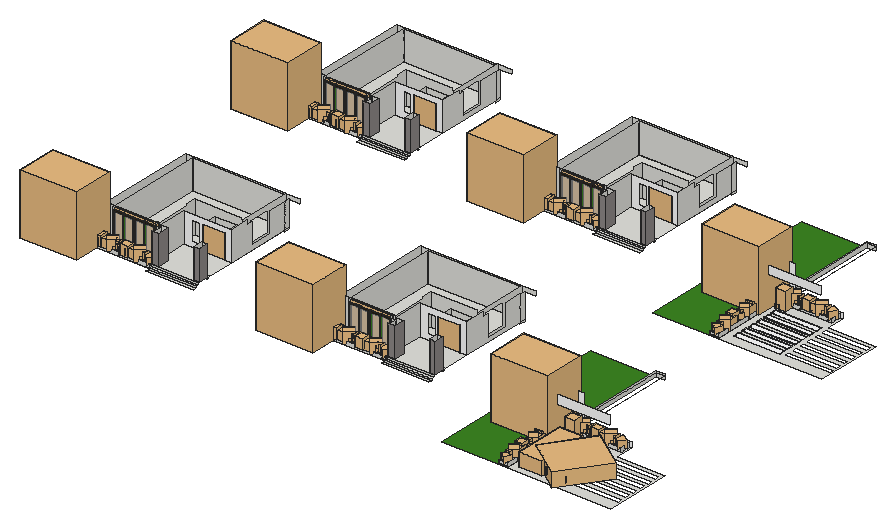
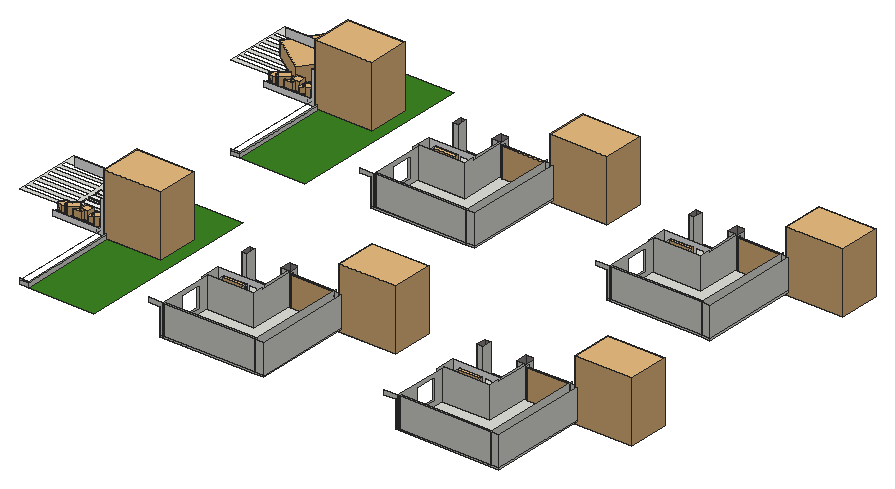
# SketchUp Ruby script. Lengths in inches.
U = 1.inch
M = Sketchup.active_model
def pt(a) = Geom::Point3d.new(a.map { |v| v * U })
def face(e, loops, mat)
  f = e.add_face(loops[0].map { |a| pt(a) })
  loops[1..].each { |l| e.add_face(l.map { |a| pt(a) }).erase! }
  f.material = f.back_material = mat if mat
  f
end
# faces: each face lists its corners as indices into pts; further lists are holes
def faces(e, pts, list, mat = nil) = list.each { |f| face(e, (f[0].is_a?(Array) ? f : [f]).map { |l| l.map { |i| pts[i] } }, mat) }
# xy, xz, yz: faces in a plane at the given z, y or x. An outline is a flat list of corners, or four numbers for a rectangle; further outlines are holes
def ring(l) = l.size == 4 ? [[l[0], l[1]], [l[2], l[1]], [l[2], l[3]], [l[0], l[3]]] : l.each_slice(2).to_a
def flat(e, list, mat, &to3) = list.each { |f| face(e, (f[0].is_a?(Array) ? f : [f]).map { |l| ring(l).map { |u, v| to3.(u, v) } }, mat) }
def xy(e, z, list, mat = nil) = flat(e, list, mat) { |x, y| [x, y, z] }
def xz(e, y, list, mat = nil) = flat(e, list, mat) { |x, z| [x, y, z] }
def yz(e, x, list, mat = nil) = flat(e, list, mat) { |y, z| [x, y, z] }
def lines(e, pts, list) = list.each { |a, b| e.add_line(pt(pts[a]), pt(pts[b])) }
# prism: a flat outline (further loops are holes) pulled along v
def prism(e, loops, v, mat = nil)
  f = face(e, loops, mat); d = Geom::Vector3d.new(v.map { |x| x * U })
  f.pushpull(f.normal.samedirection?(d) ? d.length : -d.length)
end
def box(e, o, s, mat = nil) = prism(e, [[o, [o[0] + s[0], o[1], o[2]], [o[0] + s[0], o[1] + s[1], o[2]], [o[0], o[1] + s[1], o[2]]]], [0, 0, s[2]], mat)
def at(x, y, z, deg = 0) = Geom::Transformation.translation(pt([x, y, z])) * Geom::Transformation.rotation(ORIGIN, Z_AXIS, deg.degrees)
def axes(o, x, y, z) = Geom::Transformation.new([*x, 0, *y, 0, *z, 0, *pt(o).to_a, 1])
def part(name) = M.definitions.add(name)
# library, detail: a bought-in or finely detailed component or shape, given as its bounding box
def library(name, o, s) = part(name).tap { |d| box(d.entities, o, s) }
def detail(e, o, s) = box(e.add_group.entities, o, s)
def put(e, d, t, mat = nil) = e.add_instance(d, t).tap { |i| i.material = mat if mat }
def group(e, t, mat = nil) = e.add_group.tap { |g| g.transformation = t; g.material = mat if mat }.entities
root = M.entities
M.materials.add("Material__1").color = [95, 70, 46]
M.materials.add("[Carrera Marble]").color = [255, 255, 255]
M.materials.add("[Color M00]").color = [255, 255, 255]
M.materials.add("[Color M04]").color = [60, 133, 34]
M.materials.add("[Stone Marble]1").color = [143, 138, 136]
M.materials.add("[Translucent Glass Gray]2").color = [201, 201, 201]
M.materials["[Translucent Glass Gray]2"].alpha = 0.5
M.materials.add("[Wood Veneer 01]").color = [76, 44, 23]
M.materials.add("oak swatch").color = [40, 31, 19]
c1 = library("Group\#18",[0,0,0],[68.35,49.34,73.02])
c2 = library("Areca palm plant",[0,0,0],[49.1,36.6,54.46])
c3 = library("Group\#14",[-84.69,-90.07,-0.36],[176.51,175.13,171.4])
c4 = part("Group\#15")
xy(c4.entities,0,[[0,0,6,234.8],[30,0,36,234.8]])
xy(c4.entities,3,[[6,0,30,234.8]])
xy(c4.entities,7,[[6,5,30,229.8]],"Material__1")
xy(c4.entities,15,[[[0,0,36,234.8],[6,5,30,229.8]]])
xz(c4.entities,0,[[0,0,6,0,6,3,30,3,30,0,36,0,36,15,0,15]])
xz(c4.entities,5,[[6,7,30,15]])
xz(c4.entities,229.8,[[6,7,30,15]])
xz(c4.entities,234.8,[[0,0,0,15,36,15,36,0,30,0,30,3,6,3,6,0]])
yz(c4.entities,0,[[0,0,234.8,15]])
yz(c4.entities,6,[[0,0,234.8,3],[5,7,229.8,15]])
yz(c4.entities,30,[[0,0,234.8,3],[5,7,229.8,15]])
yz(c4.entities,36,[[0,0,234.8,15]])
c5 = library("Group20\#1",[-20.81,-17.08,3.79],[39.86,39.43,37.51])
c6 = library("Group38\#2",[14.01,28.44,-23.43],[18.58,18.32,38.89])
c7 = library("Group\#130",[-7.34,-1.2,0],[38.67,35.81,49.04])
c8 = part("Group\#16")
put(c8.entities,c2,axes([-6.2,158.41,6.08],[0.45017,-0.56191,0],[0.66137,0.52986,0],[0,0,0.72]))
put(c8.entities,c2,axes([-6.2,56.6,6.08],[0.45017,-0.56191,0],[0.66137,0.52986,0],[0,0,0.72]))
put(c8.entities,c3,axes([14.93,91.37,6.05],[-0.04961,-0.08593,0],[0.08593,-0.04961,0],[0,0,0.10522]))
put(c8.entities,c3,axes([14.93,145.87,6.05],[-0.04961,-0.08593,0],[0.08593,-0.04961,0],[0,0,0.10522]))
put(c8.entities,c3,axes([17.19,223.04,6.07],[-0.08133,-0.14087,0],[0.14087,-0.08133,0],[0,0,0.1725]))
put(c8.entities,c4,at(0,0,0))
put(c8.entities,c3,axes([14.93,193.18,6.05],[-0.04961,-0.08593,0],[0.08593,-0.04961,0],[0,0,0.10522]))
put(c8.entities,c3,axes([17.19,15.79,6.07],[-0.08133,-0.14087,0],[0.14087,-0.08133,0],[0,0,0.1725]))
put(c8.entities,c5,axes([18.97,181.79,4.77],[0,0.85,0],[-0.85,0,0],[0,0,0.85]))
put(c8.entities,c5,axes([18.97,79.98,4.77],[0,0.85,0],[-0.85,0,0],[0,0,0.85]))
put(c8.entities,c6,axes([-4.1,-1.15,28.17],[0.8848,0,0],[0,0.94674,0],[0,0,0.85826]))
put(c8.entities,c6,axes([-4.1,100.66,28.17],[0.8848,0,0],[0,0.94674,0],[0,0,0.85826]))
put(c8.entities,c7,axes([24.9375,89.91,8],[0,0.79,0],[-0.79,0,0],[0,0,0.79]))
put(c8.entities,c3,axes([14.93,173.12,6.05],[-0.04961,-0.08593,0],[0.08593,-0.04961,0],[0,0,0.10522]))
put(c8.entities,c3,axes([14.93,44.05,6.05],[-0.04961,-0.08593,0],[0.08593,-0.04961,0],[0,0,0.10522]))
put(c8.entities,c3,axes([14.93,71.3,6.05],[-0.04961,-0.08593,0],[0.08593,-0.04961,0],[0,0,0.10522]))
put(c8.entities,c7,axes([24.9375,191.72,8],[0,0.79,0],[-0.79,0,0],[0,0,0.79]))
put(c8.entities,c3,axes([17.19,121.23,6.07],[-0.08133,-0.14087,0],[0.14087,-0.08133,0],[0,0,0.1725]))
c9 = library("Curtains",[0,0,0],[121.73,8.19,117.22])
c10 = part("Group\#6")
box(c10.entities,[0,0,0],[1.77,4.72,80.31],"oak swatch")
c11 = part("Exterior Sliding Doors")
xy(c11.entities,0,[[1.77,33.07,3.54,70.87],[1.77,70.87,3.54,108.66]])
xy(c11.entities,0,[[0,0,1.77,33.07],[0,108.66,1.77,141.73]],"oak swatch")
xy(c11.entities,4.72,[[0,4.72,1.77,33.07],[1.77,37.8,3.54,66.14],[1.77,75.88,3.54,103.9375],[0,108.66,1.77,137.01]],"oak swatch")
xy(c11.entities,75.59,[[1.77,37.8,3.54,66.14],[1.77,75.88,3.54,103.9375]])
xy(c11.entities,75.59,[[0,4.72,1.77,33.07],[0,108.66,1.77,137.01]],"oak swatch")
xy(c11.entities,80.31,[[0,0,1.77,33.07],[1.77,33.07,3.54,70.87],[1.77,70.87,3.54,108.66],[0,108.66,1.77,141.73]],"oak swatch")
xz(c11.entities,0,[[0,0,1.77,80.31]],"oak swatch")
xz(c11.entities,4.72,[[0,4.72,1.77,75.59]],"oak swatch")
xz(c11.entities,33.07,[[0,0,1.77,4.72],[1.77,0,3.54,80.31],[0,75.59,1.77,80.31]],"oak swatch")
xz(c11.entities,37.8,[[1.77,4.72,3.54,75.59]])
xz(c11.entities,66.14,[[1.77,4.72,3.54,75.59]],"oak swatch")
xz(c11.entities,70.87,[[1.77,0,3.54,80.31]])
xz(c11.entities,75.88,[[1.77,4.72,3.54,75.59]])
xz(c11.entities,103.9375,[[1.77,4.72,3.54,75.59]],"oak swatch")
xz(c11.entities,108.66,[[1.77,4.72,3.54,75.59]])
xz(c11.entities,108.66,[[0,0,3.54,4.72],[0,75.59,3.54,80.31]],"oak swatch")
xz(c11.entities,137.01,[[0,4.72,1.77,75.59]],"oak swatch")
xz(c11.entities,141.73,[[0,0,1.77,80.31]],"oak swatch")
yz(c11.entities,0,[[0,0,33.07,0,33.07,4.72,4.72,4.72,4.72,75.59,33.07,75.59,33.07,80.31,0,80.31],[108.66,0,141.73,0,141.73,80.31,108.66,80.31,108.66,75.59,137.01,75.59,137.01,4.72,108.66,4.72]],"oak swatch")
yz(c11.entities,1.77,[[4.72,4.72,33.07,75.59],[37.8,4.72,66.14,75.59],[75.88,4.72,103.9375,75.59],[108.66,4.72,137.01,75.59]],"[Translucent Glass Gray]2")
yz(c11.entities,1.77,[[0,0,33.07,0,33.07,4.72,4.72,4.72,4.72,75.59,33.07,75.59,33.07,80.31,0,80.31],[[33.07,0,70.87,80.31],[37.8,4.72,66.14,75.59]],[[70.87,0,141.73,80.31],[108.66,4.72,137.01,75.59],[75.88,4.72,103.9375,75.59]]],"oak swatch")
yz(c11.entities,3.54,[[[33.07,0,70.87,80.31],[37.8,4.72,66.14,75.59]],[[70.87,0,108.66,80.31],[75.88,4.72,103.9375,75.59]]],"oak swatch")
put(c11.entities,c10,at(0,33.07,0))
put(c11.entities,c10,at(0,103.9375,0))
c12 = library("modern+door",[0,0,0],[59.06,11.8125,86.61])
c13 = part("Group\#17")
put(c13.entities,c2,axes([-6.2,56.6,6.08],[0.45017,-0.56191,0],[0.66137,0.52986,0],[0,0,0.72]))
put(c13.entities,c2,axes([-6.2,158.41,6.08],[0.45017,-0.56191,0],[0.66137,0.52986,0],[0,0,0.72]))
put(c13.entities,c3,axes([14.93,44.05,6.05],[-0.04961,-0.08593,0],[0.08593,-0.04961,0],[0,0,0.10522]))
put(c13.entities,c3,axes([14.93,71.3,6.05],[-0.04961,-0.08593,0],[0.08593,-0.04961,0],[0,0,0.10522]))
put(c13.entities,c5,axes([18.97,79.98,4.77],[0,0.85,0],[-0.85,0,0],[0,0,0.85]))
put(c13.entities,c3,axes([14.93,145.87,6.05],[-0.04961,-0.08593,0],[0.08593,-0.04961,0],[0,0,0.10522]))
put(c13.entities,c3,axes([17.19,15.79,6.07],[-0.08133,-0.14087,0],[0.14087,-0.08133,0],[0,0,0.1725]))
put(c13.entities,c3,axes([17.19,223.04,6.07],[-0.08133,-0.14087,0],[0.14087,-0.08133,0],[0,0,0.1725]))
put(c13.entities,c3,axes([17.19,121.23,6.07],[-0.08133,-0.14087,0],[0.14087,-0.08133,0],[0,0,0.1725]))
put(c13.entities,c7,axes([24.9375,191.72,8],[0,0.79,0],[-0.79,0,0],[0,0,0.79]))
put(c13.entities,c7,axes([24.9375,89.91,8],[0,0.79,0],[-0.79,0,0],[0,0,0.79]))
put(c13.entities,c3,axes([14.93,91.37,6.05],[-0.04961,-0.08593,0],[0.08593,-0.04961,0],[0,0,0.10522]))
put(c13.entities,c5,axes([18.97,181.79,4.77],[0,0.85,0],[-0.85,0,0],[0,0,0.85]))
put(c13.entities,c6,axes([-4.1,-1.15,28.17],[0.8848,0,0],[0,0.94674,0],[0,0,0.85826]))
put(c13.entities,c6,axes([-4.1,100.66,28.17],[0.8848,0,0],[0,0.94674,0],[0,0,0.85826]))
put(c13.entities,c4,at(0,0,0))
put(c13.entities,c3,axes([14.93,173.12,6.05],[-0.04961,-0.08593,0],[0.08593,-0.04961,0],[0,0,0.10522]))
put(c13.entities,c3,axes([14.93,193.18,6.05],[-0.04961,-0.08593,0],[0.08593,-0.04961,0],[0,0,0.10522]))
c14 = library("Plant",[0,0,0],[12.59,12.59,14.16])
c15 = library("plant1",[-367.84,-375.82,-125.45],[750.59,696.16,1346.74])
c16 = part("skp4FF")
put(c16.entities,c15,at(0,0,0))
c17 = library("BMW 8 Series M850i 2019",[-14.25,0.77,-0.16],[87.38,190.63,50.87])
c18 = library("Omni Light",[-12,-12,-12],[24,24,24])
c19 = library("Omni Light\#1",[-12,-12,-12],[24,24,24])
c20 = library("002+Bmw+M4+++mat3.4+2017",[-252.8,19.48,9.01],[196.94,171.32,55.15])
c21 = library("Omni Light\#2",[-12,-12,-12],[24,24,24])
c22 = library("Omni Light\#3",[-12,-12,-12],[24,24,24])
xy(root,-14.85,[[[2064.92,315.5,2456.54,315.5,2456.54,568.0625,2276.89,568.0625,2276.89,636.6875,2064.92,636.6875,2064.92,593.125,2037.92,593.125,2037.92,586.4375,2064.92,586.4375],[2090.64,356.98,2264.14,378.48],[2279.14,532.29,2452.64,553.79],[2279.14,497.23,2452.64,518.73],[2279.14,462.17,2452.64,483.67],[2279.14,427.11,2452.64,448.61],[2279.14,392.04,2452.64,413.54],[2279.14,356.98,2452.64,378.48],[2090.64,532.29,2264.14,553.79],[2090.64,497.23,2264.14,518.73],[2090.64,462.17,2264.14,483.67],[2090.64,427.11,2264.14,448.61],[2090.64,392.04,2264.14,413.54]],[2037.92,536.1875,2064.92,586.4375],[[2064.92,1314.85,2456.54,1314.85,2456.54,1567.42,2276.89,1567.42,2276.89,1636.04,2064.92,1636.04,2064.92,1592.48,2037.92,1592.48,2037.92,1585.79,2064.92,1585.79],[2279.14,1531.65,2452.64,1553.15],[2279.14,1496.59,2452.64,1518.09],[2279.14,1461.52,2452.64,1483.02],[2279.14,1426.46,2452.64,1447.96],[2279.14,1391.4,2452.64,1412.9],[2279.14,1356.34,2452.64,1377.84],[2090.64,1531.65,2264.14,1553.15],[2090.64,1496.59,2264.14,1518.09],[2090.64,1461.52,2264.14,1483.02],[2090.64,1426.46,2264.14,1447.96],[2090.64,1391.4,2264.14,1412.9],[2090.64,1356.34,2264.14,1377.84]],[2037.92,1535.54,2064.92,1585.79]])
xy(root,-14.85,[[[1815.63,315.5,2037.92,315.5,2037.92,593.125,2064.92,593.125,2064.92,1019,1815.63,1019],[1959.19,562.6,1962.35,565.76,1962.35,562.6]],[1959.19,562.6,1962.35,562.6,1962.35,565.76],[[1815.63,1314.85,2037.92,1314.85,2037.92,1592.48,2064.92,1592.48,2064.92,2018.36,1815.63,2018.36],[1959.19,1561.96,1962.35,1565.12,1962.35,1561.96]],[1959.19,1561.96,1962.35,1561.96,1962.35,1565.12]],"[Color M04]")
xy(root,-14.85,[[2037.92,315.5,2064.92,536.1875],[2037.92,1314.85,2064.92,1535.54]],"[Wood Veneer 01]")
xy(root,-13.54,[[2090.64,356.98,2264.14,378.48],[2090.64,392.04,2264.14,413.54],[2090.64,427.11,2264.14,448.61],[2090.64,462.17,2264.14,483.67],[2090.64,497.23,2264.14,518.73],
  [2090.64,532.29,2264.14,553.79],[2090.64,1356.34,2264.14,1377.84],[2090.64,1391.4,2264.14,1412.9],[2090.64,1426.46,2264.14,1447.96],[2090.64,1461.52,2264.14,1483.02],
  [2090.64,1496.59,2264.14,1518.09],[2090.64,1531.65,2264.14,1553.15]],"[Carrera Marble]")
xy(root,-11.11,[[491.71,570.37,671.36,582.24],[1384.3,570.37,1563.95,582.24],[491.71,1569.72,671.36,1581.6],[1384.3,1569.72,1563.95,1581.6]])
xy(root,-4.74,[[491.71,582.24,671.36,592.87],[1384.3,582.24,1563.95,592.87],[491.71,1581.6,671.36,1592.22],[1384.3,1581.6,1563.95,1592.22]])
xy(root,1.3125,[[491.71,592.87,519.14,597.99],[519.14,592.87,649.86,592.87,649.86,635.56,671.36,635.56,671.36,749.87,645.68,749.87,645.68,808.37,561.42,808.37,561.42,749.87,491.71,749.87,491.71,638.93,519.14,638.93],[649.86,592.87,671.36,597.99],[1384.3,592.87,1411.73,597.99],[1411.73,592.87,1542.45,592.87,1542.45,635.56,1563.95,635.56,1563.95,749.87,1538.27,749.87,1538.27,808.37,1454.01,808.37,1454.01,749.87,1384.3,749.87,1384.3,638.93,1411.73,638.93],
  [1542.45,592.87,1563.95,597.99],[491.71,597.99,519.14,638.93],[649.86,597.99,671.36,635.56],[1384.3,597.99,1411.73,638.93],[1542.45,597.99,1563.95,635.56],
  [312.05,638.99,472.88,648.22],[472.88,638.99,491.71,648.22],[1204.64,638.99,1365.47,648.22],[1365.47,638.99,1384.3,648.22],[279.74,648.22,312.05,1021.31],
  [312.05,648.22,481.36,648.22,481.36,813.85,662.14,813.85,662.14,1021.31,655.66,1021.31,655.66,1013.93,312.05,1013.93],[481.36,648.22,491.71,648.22,491.71,749.87,561.42,749.87,561.42,808.37,645.68,808.37,645.68,749.87,662.14,749.87,662.14,813.85,481.36,813.85],[1172.33,648.22,1204.64,1021.31],[1204.64,648.22,1373.95,648.22,1373.95,813.85,1554.73,813.85,1554.73,1021.31,1548.25,1021.31,1548.25,1013.93,1204.64,1013.93],[1373.95,648.22,1384.3,648.22,1384.3,749.87,1454.01,749.87,1454.01,808.37,1538.27,808.37,1538.27,749.87,1554.73,749.87,1554.73,813.85,1373.95,813.85],
  [662.14,749.87,671.36,1021.31],[1554.73,749.87,1563.95,1021.31],[312.05,1013.93,655.66,1021.31],[1204.64,1013.93,1548.25,1021.31],[491.71,1592.22,519.14,1597.35],
  [519.14,1592.22,649.86,1592.22,649.86,1634.91,671.36,1634.91,671.36,1749.22,645.68,1749.22,645.68,1807.72,561.42,1807.72,561.42,1749.22,491.71,1749.22,491.71,1638.29,519.14,1638.29],[649.86,1592.22,671.36,1597.35],[1384.3,1592.22,1411.73,1597.35],[1411.73,1592.22,1542.45,1592.22,1542.45,1634.91,1563.95,1634.91,1563.95,1749.22,1538.27,1749.22,1538.27,1807.72,1454.01,1807.72,1454.01,1749.22,1384.3,1749.22,1384.3,1638.29,1411.73,1638.29],[1542.45,1592.22,1563.95,1597.35],
  [491.71,1597.35,519.14,1638.29],[649.86,1597.35,671.36,1634.91],[1384.3,1597.35,1411.73,1638.29],[1542.45,1597.35,1563.95,1634.91],[312.05,1638.35,472.88,1647.57],
  [472.88,1638.35,491.71,1647.57],[1204.64,1638.35,1365.47,1647.57],[1365.47,1638.35,1384.3,1647.57],[279.74,1647.57,312.05,2020.66],[312.05,1647.57,481.36,1647.57,481.36,1813.21,662.14,1813.21,662.14,2020.66,655.66,2020.66,655.66,2013.29,312.05,2013.29],
  [481.36,1647.57,491.71,1647.57,491.71,1749.22,561.42,1749.22,561.42,1807.72,645.68,1807.72,645.68,1749.22,662.14,1749.22,662.14,1813.21,481.36,1813.21],[1172.33,1647.57,1204.64,2020.66],[1204.64,1647.57,1373.95,1647.57,1373.95,1813.21,1554.73,1813.21,1554.73,2020.66,1548.25,2020.66,1548.25,2013.29,1204.64,2013.29],[1373.95,1647.57,1384.3,1647.57,1384.3,1749.22,1454.01,1749.22,1454.01,1807.72,1538.27,1807.72,1538.27,1749.22,1554.73,1749.22,1554.73,1813.21,1373.95,1813.21],[662.14,1749.22,671.36,2020.66],
  [1554.73,1749.22,1563.95,2020.66],[312.05,2013.29,655.66,2020.66],[1204.64,2013.29,1548.25,2020.66]])
xz(root,356.98,[[2090.64,-14.85,2264.14,-13.54]])
xz(root,378.48,[[2090.64,-14.85,2264.14,-13.54]])
xz(root,392.04,[[2090.64,-14.85,2264.14,-13.54]])
xz(root,413.54,[[2090.64,-14.85,2264.14,-13.54]])
xz(root,427.11,[[2090.64,-14.85,2264.14,-13.54]])
xz(root,448.61,[[2090.64,-14.85,2264.14,-13.54]])
xz(root,462.17,[[2090.64,-14.85,2264.14,-13.54]])
xz(root,483.67,[[2090.64,-14.85,2264.14,-13.54]])
xz(root,497.23,[[2090.64,-14.85,2264.14,-13.54]])
xz(root,518.73,[[2090.64,-14.85,2264.14,-13.54]])
xz(root,532.29,[[2090.64,-14.85,2264.14,-13.54]])
xz(root,536.1875,[[2037.92,-14.85,2064.92,-14.85,2064.92,109.625,2276.89,109.625,2276.89,142.875,2037.92,142.875]],"[Color M00]")
xz(root,553.79,[[2090.64,-14.85,2264.14,-13.54]])
xz(root,582.24,[[491.71,-11.11,671.36,-4.74],[1384.3,-11.11,1563.95,-4.74]])
xz(root,586.4375,[[2037.92,-14.85,2064.92,109.5]])
xz(root,592.87,[[491.71,-4.74,671.36,1.3125],[1384.3,-4.74,1563.95,1.3125]])
xz(root,597.99,[[491.71,1.3125,519.14,113.8125],[649.86,1.3125,671.36,113.8125],[1384.3,1.3125,1411.73,113.8125],[1542.45,1.3125,1563.95,113.8125]],"[Stone Marble]1")
xz(root,635.56,[[649.86,1.3125,671.36,113.8125],[1542.45,1.3125,1563.95,113.8125]])
xz(root,636.6875,[[2064.92,-14.85,2276.89,-14.85,2276.89,6,2097.23,6,2097.23,109.5,2064.92,109.5]],"[Color M00]")
xz(root,638.93,[[491.71,1.3125,519.14,113.8125],[1384.3,1.3125,1411.73,113.8125]])
xz(root,638.99,[[491.71,-4.74,671.36,-4.6875],[1384.3,-4.74,1563.95,-4.6875],[472.88,1.3125,491.71,104.9375],[1365.47,1.3125,1384.3,104.9375]])
xz(root,648.22,[[294.49,1.3125,312.05,113.8125],[472.88,1.3125,481.36,113.8125],[1187.08,1.3125,1204.64,113.8125],[1365.47,1.3125,1373.95,113.8125]])
xz(root,749.87,[[[491.71,1.3125,561.42,1.3125,561.42,93.27,645.68,93.27,645.68,1.3125,671.36,1.3125,671.36,113.8125,491.71,113.8125],[523.18,21.58,552.96,93.3]],[[1384.3,1.3125,1454.01,1.3125,1454.01,93.27,1538.27,93.27,1538.27,1.3125,1563.95,1.3125,1563.95,113.8125,1384.3,113.8125],[1415.77,21.58,1445.55,93.3]]],"[Color M00]")
xz(root,808.37,[[561.42,1.3125,645.68,93.27],[1454.01,1.3125,1538.27,93.27]])
xz(root,813.85,[[481.36,1.3125,481.36,121.3125,655.66,121.3125,655.66,113.8125,662.14,113.8125,662.14,1.3125],[1373.95,1.3125,1373.95,121.3125,1548.25,121.3125,1548.25,113.8125,1554.73,113.8125,1554.73,1.3125]])
xz(root,1013.93,[[312.05,1.3125,655.66,113.8125],[1204.64,1.3125,1548.25,113.8125]])
xz(root,1019,[[2064.92,-14.85,2097.23,0],[2064.92,0,2097.23,6]])
xz(root,1021.31,[[279.74,-4.6875,312.05,1.3125],[312.05,-4.6875,671.36,1.3125],[1172.33,-4.6875,1204.64,1.3125],[1204.64,-4.6875,1563.95,1.3125],[279.74,1.3125,312.05,113.8125],
  [312.05,1.3125,655.66,113.8125],[655.66,1.3125,662.14,113.8125],[662.14,1.3125,662.14,113.8125,715.11,113.8125,715.11,97.9375,671.36,97.9375,671.36,1.3125],[1172.33,1.3125,1204.64,113.8125],[1204.64,1.3125,1548.25,113.8125],
  [1548.25,1.3125,1554.73,113.8125],[1554.73,1.3125,1554.73,113.8125,1607.7,113.8125,1607.7,97.9375,1563.95,97.9375,1563.95,1.3125]])
xz(root,1356.34,[[2090.64,-14.85,2264.14,-13.54]])
xz(root,1377.84,[[2090.64,-14.85,2264.14,-13.54]])
xz(root,1391.4,[[2090.64,-14.85,2264.14,-13.54]])
xz(root,1412.9,[[2090.64,-14.85,2264.14,-13.54]])
xz(root,1426.46,[[2090.64,-14.85,2264.14,-13.54]])
xz(root,1447.96,[[2090.64,-14.85,2264.14,-13.54]])
xz(root,1461.52,[[2090.64,-14.85,2264.14,-13.54]])
xz(root,1483.02,[[2090.64,-14.85,2264.14,-13.54]])
xz(root,1496.59,[[2090.64,-14.85,2264.14,-13.54]])
xz(root,1518.09,[[2090.64,-14.85,2264.14,-13.54]])
xz(root,1531.65,[[2090.64,-14.85,2264.14,-13.54]])
xz(root,1535.54,[[2037.92,-14.85,2064.92,-14.85,2064.92,109.625,2276.89,109.625,2276.89,142.875,2037.92,142.875]],"[Color M00]")
xz(root,1553.15,[[2090.64,-14.85,2264.14,-13.54]])
xz(root,1581.6,[[491.71,-11.11,671.36,-4.74],[1384.3,-11.11,1563.95,-4.74]])
xz(root,1585.79,[[2037.92,-14.85,2064.92,109.5]])
xz(root,1592.22,[[491.71,-4.74,671.36,1.3125],[1384.3,-4.74,1563.95,1.3125]])
xz(root,1597.35,[[491.71,1.3125,519.14,113.8125],[649.86,1.3125,671.36,113.8125],[1384.3,1.3125,1411.73,113.8125],[1542.45,1.3125,1563.95,113.8125]],"[Stone Marble]1")
xz(root,1634.91,[[649.86,1.3125,671.36,113.8125],[1542.45,1.3125,1563.95,113.8125]])
xz(root,1636.04,[[2064.92,-14.85,2276.89,-14.85,2276.89,6,2097.23,6,2097.23,109.5,2064.92,109.5]],"[Color M00]")
xz(root,1638.29,[[491.71,1.3125,519.14,113.8125],[1384.3,1.3125,1411.73,113.8125]])
xz(root,1638.35,[[491.71,-4.74,671.36,-4.6875],[1384.3,-4.74,1563.95,-4.6875],[472.88,1.3125,491.71,104.9375],[1365.47,1.3125,1384.3,104.9375]])
xz(root,1647.57,[[294.49,1.3125,312.05,113.8125],[472.88,1.3125,481.36,113.8125],[1187.08,1.3125,1204.64,113.8125],[1365.47,1.3125,1373.95,113.8125]])
xz(root,1749.22,[[[491.71,1.3125,561.42,1.3125,561.42,93.27,645.68,93.27,645.68,1.3125,671.36,1.3125,671.36,113.8125,491.71,113.8125],[523.18,21.58,552.96,93.3]],[[1384.3,1.3125,1454.01,1.3125,1454.01,93.27,1538.27,93.27,1538.27,1.3125,1563.95,1.3125,1563.95,113.8125,1384.3,113.8125],[1415.77,21.58,1445.55,93.3]]],"[Color M00]")
xz(root,1807.72,[[561.42,1.3125,645.68,93.27],[1454.01,1.3125,1538.27,93.27]])
xz(root,1813.21,[[481.36,1.3125,481.36,121.3125,655.66,121.3125,655.66,113.8125,662.14,113.8125,662.14,1.3125],[1373.95,1.3125,1373.95,121.3125,1548.25,121.3125,1548.25,113.8125,1554.73,113.8125,1554.73,1.3125]])
xz(root,2013.29,[[312.05,1.3125,655.66,113.8125],[1204.64,1.3125,1548.25,113.8125]])
xz(root,2018.36,[[2064.92,-14.85,2097.23,0],[2064.92,0,2097.23,6]])
xz(root,2020.66,[[279.74,-4.6875,312.05,1.3125],[312.05,-4.6875,671.36,1.3125],[1172.33,-4.6875,1204.64,1.3125],[1204.64,-4.6875,1563.95,1.3125],[279.74,1.3125,312.05,113.8125],
  [312.05,1.3125,655.66,113.8125],[655.66,1.3125,662.14,113.8125],[662.14,1.3125,662.14,113.8125,715.11,113.8125,715.11,97.9375,671.36,97.9375,671.36,1.3125],[1172.33,1.3125,1204.64,113.8125],[1204.64,1.3125,1548.25,113.8125],
  [1548.25,1.3125,1554.73,113.8125],[1554.73,1.3125,1554.73,113.8125,1607.7,113.8125,1607.7,97.9375,1563.95,97.9375,1563.95,1.3125]])
yz(root,279.74,[[638.99,-4.6875,1021.31,1.3125],[1638.35,-4.6875,2020.66,1.3125],[638.99,1.3125,648.22,113.8125],[648.22,1.3125,1021.31,113.8125],[1638.35,1.3125,1647.57,113.8125],
  [1647.57,1.3125,2020.66,113.8125]])
yz(root,312.05,[[638.99,1.3125,648.22,113.8125],[648.22,1.3125,1013.93,113.8125],[1013.93,1.3125,1021.31,113.8125],[1638.35,1.3125,1647.57,113.8125],[1647.57,1.3125,2013.29,113.8125],
  [2013.29,1.3125,2020.66,113.8125]])
yz(root,472.88,[[638.99,1.3125,648.22,113.8125],[1638.35,1.3125,1647.57,113.8125]])
yz(root,481.36,[[648.22,1.3125,648.22,113.8125,776.62,113.8125,776.62,121.3125,813.85,121.3125,813.85,1.3125],[1647.57,1.3125,1647.57,113.8125,1775.97,113.8125,1775.97,121.3125,1813.21,121.3125,1813.21,1.3125]])
yz(root,491.71,[[582.24,-11.11,592.87,-4.74],[592.87,-11.11,638.99,-4.74],[1581.6,-11.11,1592.22,-4.74],[1592.22,-11.11,1638.35,-4.74],[592.87,-4.74,638.99,1.3125],
  [1592.22,-4.74,1638.35,1.3125],[597.99,1.3125,638.93,104.9375],[638.99,1.3125,749.87,113.8125],[1597.35,1.3125,1638.29,104.9375],[1638.35,1.3125,1749.22,113.8125]])
yz(root,519.14,[[597.99,1.3125,638.93,113.8125],[1597.35,1.3125,1638.29,113.8125]],"[Stone Marble]1")
yz(root,561.42,[[749.87,1.3125,808.37,93.27],[1749.22,1.3125,1807.72,93.27]])
yz(root,645.68,[[749.87,1.3125,808.37,93.27],[1749.22,1.3125,1807.72,93.27]])
yz(root,649.86,[[597.99,1.3125,635.56,113.8125],[1597.35,1.3125,1634.91,113.8125]])
yz(root,655.66,[[1013.93,1.3125,1021.31,113.8125],[2013.29,1.3125,2020.66,113.8125]])
yz(root,662.14,[[[813.85,1.3125,1021.31,113.8125],[847.15,18.5,931.78,97.9375]],[[1813.21,1.3125,2020.66,113.8125],[1846.51,18.5,1931.13,97.9375]]])
yz(root,671.36,[[1001.66,-4.6875,1021.31,1.3125],[2001.02,-4.6875,2020.66,1.3125],[749.87,1.3125,1001.66,1.3125,1001.66,97.9375,931.78,97.9375,931.78,18.5,847.15,18.5,847.15,97.9375,824.85,97.9375,824.85,113.8125,749.87,113.8125],[1001.66,1.3125,1021.31,97.9375],[1749.22,1.3125,2001.02,1.3125,2001.02,97.9375,1931.13,97.9375,1931.13,18.5,1846.51,18.5,1846.51,97.9375,1824.2,97.9375,1824.2,113.8125,1749.22,113.8125],
  [2001.02,1.3125,2020.66,97.9375]])
yz(root,671.36,[[597.99,1.3125,635.56,113.8125],[1597.35,1.3125,1634.91,113.8125]],"[Stone Marble]1")
yz(root,1172.33,[[638.99,-4.6875,1021.31,1.3125],[1638.35,-4.6875,2020.66,1.3125],[638.99,1.3125,648.22,113.8125],[648.22,1.3125,1021.31,113.8125],[1638.35,1.3125,1647.57,113.8125],
  [1647.57,1.3125,2020.66,113.8125]])
yz(root,1204.64,[[638.99,1.3125,648.22,113.8125],[648.22,1.3125,1013.93,113.8125],[1013.93,1.3125,1021.31,113.8125],[1638.35,1.3125,1647.57,113.8125],[1647.57,1.3125,2013.29,113.8125],
  [2013.29,1.3125,2020.66,113.8125]])
yz(root,1365.47,[[638.99,1.3125,648.22,113.8125],[1638.35,1.3125,1647.57,113.8125]])
yz(root,1373.95,[[648.22,1.3125,648.22,113.8125,776.62,113.8125,776.62,121.3125,813.85,121.3125,813.85,1.3125],[1647.57,1.3125,1647.57,113.8125,1775.97,113.8125,1775.97,121.3125,1813.21,121.3125,1813.21,1.3125]])
yz(root,1384.3,[[582.24,-11.11,592.87,-4.74],[592.87,-11.11,638.99,-4.74],[1581.6,-11.11,1592.22,-4.74],[1592.22,-11.11,1638.35,-4.74],[592.87,-4.74,638.99,1.3125],
  [1592.22,-4.74,1638.35,1.3125],[597.99,1.3125,638.93,104.9375],[638.99,1.3125,749.87,113.8125],[1597.35,1.3125,1638.29,104.9375],[1638.35,1.3125,1749.22,113.8125]])
yz(root,1411.73,[[597.99,1.3125,638.93,113.8125],[1597.35,1.3125,1638.29,113.8125]],"[Stone Marble]1")
yz(root,1454.01,[[749.87,1.3125,808.37,93.27],[1749.22,1.3125,1807.72,93.27]])
yz(root,1538.27,[[749.87,1.3125,808.37,93.27],[1749.22,1.3125,1807.72,93.27]])
yz(root,1542.45,[[597.99,1.3125,635.56,113.8125],[1597.35,1.3125,1634.91,113.8125]])
yz(root,1548.25,[[1013.93,1.3125,1021.31,113.8125],[2013.29,1.3125,2020.66,113.8125]])
yz(root,1554.73,[[[813.85,1.3125,1021.31,113.8125],[847.15,18.5,931.78,97.9375]],[[1813.21,1.3125,2020.66,113.8125],[1846.51,18.5,1931.13,97.9375]]])
yz(root,1563.95,[[1001.66,-4.6875,1021.31,1.3125],[2001.02,-4.6875,2020.66,1.3125],[749.87,1.3125,1001.66,1.3125,1001.66,97.9375,931.78,97.9375,931.78,18.5,847.15,18.5,847.15,97.9375,824.85,97.9375,824.85,113.8125,749.87,113.8125],[1001.66,1.3125,1021.31,97.9375],[1749.22,1.3125,2001.02,1.3125,2001.02,97.9375,1931.13,97.9375,1931.13,18.5,1846.51,18.5,1846.51,97.9375,1824.2,97.9375,1824.2,113.8125,1749.22,113.8125],
  [2001.02,1.3125,2020.66,97.9375]])
yz(root,1563.95,[[597.99,1.3125,635.56,113.8125],[1597.35,1.3125,1634.91,113.8125]],"[Stone Marble]1")
yz(root,2037.92,[[536.1875,-14.85,536.1875,142.875,636.6875,142.875,636.6875,109.5,586.4375,109.5,586.4375,-14.85],[1535.54,-14.85,1535.54,142.875,1636.04,142.875,1636.04,109.5,1585.79,109.5,1585.79,-14.85]])
yz(root,2064.92,[[636.6875,-14.85,1019,0],[1636.04,-14.85,2018.36,0],[636.6875,0,1019,6],[1636.04,0,2018.36,6]])
yz(root,2064.92,[[536.1875,-14.85,586.4375,-14.85,586.4375,109.5,636.6875,109.5,636.6875,109.625,536.1875,109.625],[1535.54,-14.85,1585.79,-14.85,1585.79,109.5,1636.04,109.5,1636.04,109.625,1535.54,109.625]],"[Wood Veneer 01]")
yz(root,2090.64,[[356.98,-14.85,378.48,-13.54],[392.04,-14.85,413.54,-13.54],[427.11,-14.85,448.61,-13.54],[462.17,-14.85,483.67,-13.54],[497.23,-14.85,518.73,-13.54],
  [532.29,-14.85,553.79,-13.54],[1356.34,-14.85,1377.84,-13.54],[1391.4,-14.85,1412.9,-13.54],[1426.46,-14.85,1447.96,-13.54],[1461.52,-14.85,1483.02,-13.54],
  [1496.59,-14.85,1518.09,-13.54],[1531.65,-14.85,1553.15,-13.54]])
yz(root,2264.14,[[1356.34,-14.85,1377.84,-13.54],[1391.4,-14.85,1412.9,-13.54],[1426.46,-14.85,1447.96,-13.54],[1496.59,-14.85,1518.09,-13.54],[1531.65,-14.85,1553.15,-13.54]])
p = [[2106.46,645.91,0],[2106.46,645.91,6],[2106.46,645.91,-1.6875],[2097.23,1019,0],[2097.23,636.6875,0],[321.28,648.22,-4.6875],
  [662.14,648.22,-4.6875],[662.14,648.22,1.3125],[321.28,648.22,1.3125],[1213.87,648.22,-4.6875],[1213.87,648.22,-6.375],[321.28,648.22,-6.375],
  [662.14,648.22,-6.375],[1204.64,1021.31,-4.6875],[1204.64,638.99,-4.6875],[1554.73,648.22,-4.6875],[1554.73,648.22,-6.375],[312.05,1021.31,-4.6875],
  [312.05,638.99,-4.6875],[671.36,648.22,1.3125],[1554.73,648.22,1.3125],[1563.95,648.22,1.3125],[1213.87,648.22,1.3125],[2106.46,1645.27,0],
  [2106.46,1645.27,6],[2106.46,1645.27,-1.6875],[2097.23,2018.36,0],[2097.23,1636.04,0],[662.14,1647.57,-4.6875],[662.14,1647.57,-6.375],
  [321.28,1647.57,-4.6875],[321.28,1647.57,-6.375],[1204.64,2020.66,-4.6875],[1204.64,1638.35,-4.6875],[1554.73,1647.57,-4.6875],[1554.73,1647.57,-6.375],
  [312.05,2020.66,-4.6875],[312.05,1638.35,-4.6875],[662.14,1647.57,1.3125],[671.36,1647.57,1.3125],[1554.73,1647.57,1.3125],[1563.95,1647.57,1.3125],
  [1213.87,1647.57,-4.6875],[1213.87,1647.57,-6.375],[1213.87,1647.57,1.3125],[321.28,1647.57,1.3125]]
lines(root,p,[[0,1],[0,2],[3,4],[5,6],[6,7],[5,8],[9,10],[5,11],[6,12],[13,14],[15,16],[17,18],
  [7,19],[20,21],[15,20],[9,22],[9,15],[23,24],[23,25],[26,27],[28,29],[30,31],[32,33],[34,35],
  [36,37],[38,39],[40,41],[42,43],[34,40],[42,44],[42,34],[30,28],[28,38],[30,45]])
put(root,c1,axes([72.07,1496.56,-14],[3.16,0,0],[0,3.16,0],[0,0,3.16]))
put(root,c1,axes([72.07,497.2,-14],[3.16,0,0],[0,3.16,0],[0,0,3.16]))
put(root,c8,at(487.65,1594.61,-15.33,90))
put(root,c8,at(487.65,595.25,-15.33,90))
put(root,c9,axes([312.05,1642.11,-1.83],[1.32124,0,0],[0,1,0],[0,0,0.96546]))
put(root,c9,axes([312.05,642.75,-1.83],[1.32124,0,0],[0,1,0],[0,0,0.96546]))
put(root,c11,axes([312.05,1640.12,1.3125],[0,-1,0],[1.13475,0,0],[0,0,1.29023]),"[Color M04]")
put(root,c11,axes([312.05,640.77,1.3125],[0,-1,0],[1.13475,0,0],[0,0,1.29023]),"[Color M04]")
put(root,c12,axes([561.42,1749.22,1.3125],[1.42694,0,0],[0,1,0],[0,0,1.06174]))
put(root,c12,axes([561.42,749.87,1.3125],[1.42694,0,0],[0,1,0],[0,0,1.06174]))
put(root,c1,axes([964.66,1496.56,-14],[3.16,0,0],[0,3.16,0],[0,0,3.16]))
put(root,c1,axes([964.66,497.2,-14],[3.16,0,0],[0,3.16,0],[0,0,3.16]))
put(root,c8,at(1380.24,1594.61,-15.33,90))
put(root,c8,at(1380.24,595.25,-15.33,90))
put(root,c9,axes([1204.64,1642.11,-1.83],[1.32124,0,0],[0,1,0],[0,0,0.96546]))
put(root,c9,axes([1204.64,642.75,-1.83],[1.32124,0,0],[0,1,0],[0,0,0.96546]))
put(root,c11,axes([1204.64,1640.12,1.3125],[0,-1,0],[1.13475,0,0],[0,0,1.29023]),"[Color M04]")
put(root,c11,axes([1204.64,640.77,1.3125],[0,-1,0],[1.13475,0,0],[0,0,1.29023]),"[Color M04]")
put(root,c12,axes([1454.01,1749.22,1.3125],[1.42694,0,0],[0,1,0],[0,0,1.06174]))
put(root,c12,axes([1454.01,749.87,1.3125],[1.42694,0,0],[0,1,0],[0,0,1.06174]))
put(root,c1,axes([1857.25,1494.25,-9.3125],[3.16,0,0],[0,3.16,0],[0,0,3.16]))
put(root,c1,axes([1857.25,494.9,-9.3125],[3.16,0,0],[0,3.16,0],[0,0,3.16]))
put(root,c13,axes([2030.12,1318.59,-14.85],[0.92,0,0],[0,0.92,0],[0,0,0.92]))
put(root,c13,axes([2030.12,319.23,-14.85],[0.92,0,0],[0,0.92,0],[0,0,0.92]))
put(root,c14,at(2080.23,1563.1,-13.54))
put(root,c14,at(2080.23,563.75,-13.54))
put(root,c16,axes([2099.5,1582.8,-7.21],[0.05049,0,0],[0,0.05049,0],[0,0,0.05049]))
put(root,c16,axes([2099.5,583.44,-7.21],[0.05049,0,0],[0,0.05049,0],[0,0,0.05049]))
put(root,c17,at(2159.99,534.35,-14.69,-180))
put(root,c8,at(2272.83,1592.3,-10.64,90))
put(root,c8,at(2272.83,592.95,-10.64,90))
put(root,c18,at(2202.1875,351.6875,9.42))
put(root,c19,at(2207.35,348.46,9.36))
put(root,c20,at(2404.37,498.74,-23.86,55))
put(root,c21,at(2252.1,348.46,8.4))
put(root,c22,at(2255.24,348.46,8.4))
